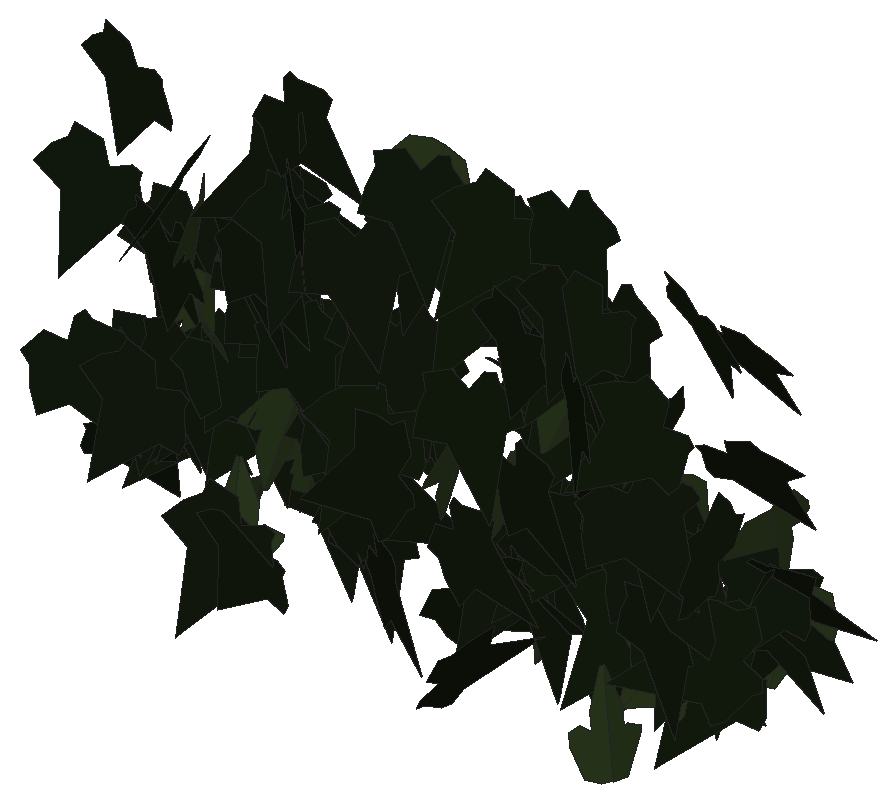
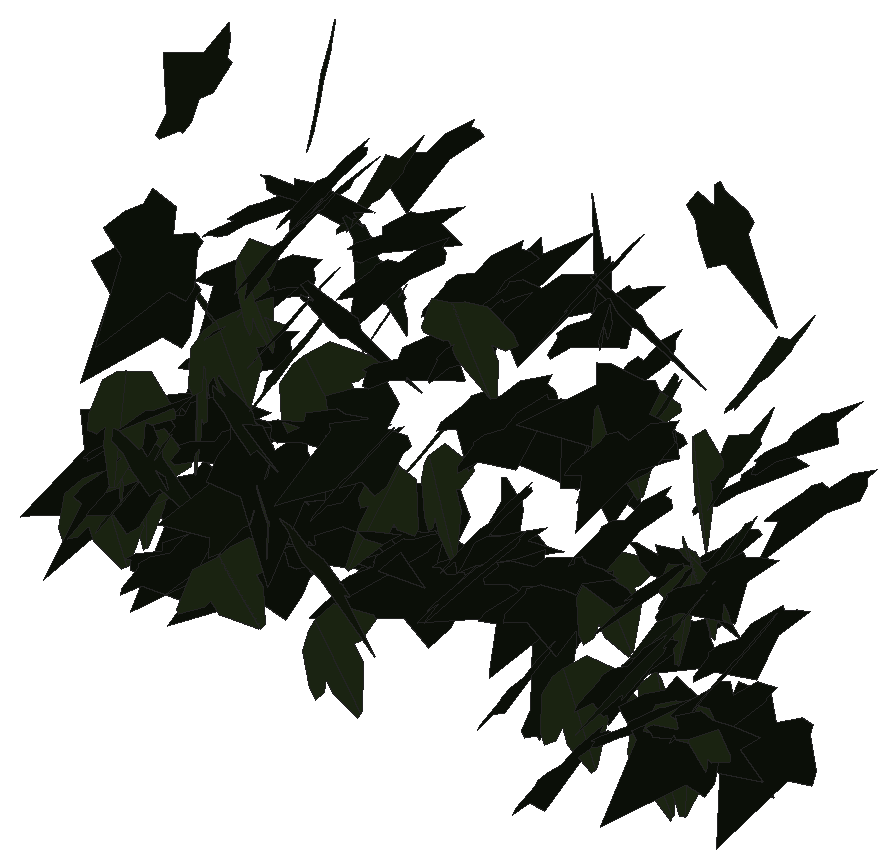
# SketchUp Ruby script. Lengths in inches.
U = 1.inch
M = Sketchup.active_model
def pt(a) = Geom::Point3d.new(a.map { |v| v * U })
def face(e, loops, mat)
  f = e.add_face(loops[0].map { |a| pt(a) })
  loops[1..].each { |l| e.add_face(l.map { |a| pt(a) }).erase! }
  f.material = f.back_material = mat if mat
  f
end
# faces: each face lists its corners as indices into pts; further lists are holes
def faces(e, pts, list, mat = nil) = list.each { |f| face(e, (f[0].is_a?(Array) ? f : [f]).map { |l| l.map { |i| pts[i] } }, mat) }
# xy, xz, yz: faces in a plane at the given z, y or x. An outline is a flat list of corners, or four numbers for a rectangle; further outlines are holes
def ring(l) = l.size == 4 ? [[l[0], l[1]], [l[2], l[1]], [l[2], l[3]], [l[0], l[3]]] : l.each_slice(2).to_a
def flat(e, list, mat, &to3) = list.each { |f| face(e, (f[0].is_a?(Array) ? f : [f]).map { |l| ring(l).map { |u, v| to3.(u, v) } }, mat) }
def xy(e, z, list, mat = nil) = flat(e, list, mat) { |x, y| [x, y, z] }
def xz(e, y, list, mat = nil) = flat(e, list, mat) { |x, z| [x, y, z] }
def yz(e, x, list, mat = nil) = flat(e, list, mat) { |y, z| [x, y, z] }
def lines(e, pts, list) = list.each { |a, b| e.add_line(pt(pts[a]), pt(pts[b])) }
# prism: a flat outline (further loops are holes) pulled along v
def prism(e, loops, v, mat = nil)
  f = face(e, loops, mat); d = Geom::Vector3d.new(v.map { |x| x * U })
  f.pushpull(f.normal.samedirection?(d) ? d.length : -d.length)
end
def box(e, o, s, mat = nil) = prism(e, [[o, [o[0] + s[0], o[1], o[2]], [o[0] + s[0], o[1] + s[1], o[2]], [o[0], o[1] + s[1], o[2]]]], [0, 0, s[2]], mat)
def at(x, y, z, deg = 0) = Geom::Transformation.translation(pt([x, y, z])) * Geom::Transformation.rotation(ORIGIN, Z_AXIS, deg.degrees)
def axes(o, x, y, z) = Geom::Transformation.new([*x, 0, *y, 0, *z, 0, *pt(o).to_a, 1])
def part(name) = M.definitions.add(name)
# library, detail: a bought-in or finely detailed component or shape, given as its bounding box
def library(name, o, s) = part(name).tap { |d| box(d.entities, o, s) }
def detail(e, o, s) = box(e.add_group.entities, o, s)
def put(e, d, t, mat = nil) = e.add_instance(d, t).tap { |i| i.material = mat if mat }
def group(e, t, mat = nil) = e.add_group.tap { |g| g.transformation = t; g.material = mat if mat }.entities
root = M.entities
M.materials.add("efeu1").color = [18, 25, 13]
M.materials.add("efeu2").color = [43, 57, 29]
c1 = part("ivyleaf_9")
p = [[1.54,2.16,1.25],[1.36,2.04,1.19],[-0.21,0.99,0.68],[-0.71,1.11,0.82],[-0.85,0.86,0.67],[-0.8,0.17,0.21],
  [-0.9,-0.01,0.1],[-0.67,-0.16,-0.02],[-0.08,-0.08,-0.05],[-0.03,-0.6,-0.4],[0.65,-0.88,-0.66],[0.83,-0.6,-0.49],
  [1.29,-0.42,-0.43],[1.8125,-0.07,-0.26],[1.21,0.44,0.15]]
faces(c1.entities,p,[[0,1,2,3,4,5,6,7,8,9,10,11,12,13,14]],"efeu1")
c2 = part("ivyleaf_10")
p = [[0,0.5,-0.03],[-0.0625,2.02,-0.43],[-0.19,2.01,-0.46],[-0.54,1.05,-0.29],[-0.52,0.625,-0.18],[-0.83,0.76,-0.28],
  [-1.16,0.64,-0.33],[-1.15,0.33,-0.24],[-0.77,-0.39,0.02],[-0.3,-0.51,0.16],[0.04,-0.48,0.23],[-0.02,2.01,-0.4375],
  [-0.06,2.01,-0.43],[0.04,-0.49,0.23],[0.67,-0.49,0.14],[1.38,0.36,-0.2],[1.375,0.51,-0.24],[0.81,0.65,-0.19],
  [0.62,0.59,-0.15],[0.6,1.09,-0.28],[0.5,1.23,-0.31]]
faces(c2.entities,p,[[0,1,2,3,4,5,6,7,8,9,10],[11,12,0,13,14,15,16,17,18,19,20]],"efeu2")
put(root,c1,axes([29.21,220.93,249.09],[0.38995,0.30515,-0.06943],[-0.05603,-0.04106,-0.49515],[-0.30789,0.39395,0.00217]))
put(root,c1,axes([29.23,220.59,252.55],[-0.16358,-0.44301,0.16426],[-0.00318,-0.17279,-0.46919],[0.47247,-0.15454,0.05372]))
put(root,c1,axes([29.22,221.13,253.58],[-0.03475,-0.39781,0.3009],[0.08116,-0.30212,-0.39005],[0.49214,0.02173,0.08557]))
put(root,c1,axes([29.36,221.97,251.31],[-0.15964,-0.47334,0.02147],[-0.00888,-0.01966,-0.49953],[0.47375,-0.15987,-0.00213]))
put(root,c1,axes([29.66,221.94,249.32],[-0.4551,-0.20171,0.04684],[-0.04917,-0.00462,-0.49756],[0.20116,-0.45748,-0.01563]))
put(root,c2,axes([29.69,221.88,249.35],[-0.49291,0.00458,0.08381],[-0.08393,-0.02123,-0.49245],[-0.00095,-0.49953,0.0217]))
put(root,c1,axes([29.5,221.12,250.18],[-0.07345,-0.49439,0.01348],[-0.0043,-0.01299,-0.49981],[0.49456,-0.07354,-0.00234]))
put(root,c1,axes([29.4,221.29,250.07],[0.20532,-0.45347,-0.04697],[-0.00661,0.04855,-0.49759],[0.45585,0.20495,0.01394]))
put(root,c1,axes([29.46,221.38,249.5625],[0.14125,-0.2738,-0.39381],[-0.04334,0.40156,-0.29473],[0.47767,0.1174,0.08971]))
put(root,c1,axes([29.46,221.49,251.3125],[0.2592,-0.42737,-0.01299],[-0.00599,0.01156,-0.49983],[0.42752,0.25927,0.00088]))
put(root,c1,axes([29.68,221.79,249.27],[0.47958,0.1413,0.00649],[-0.00505,0.04001,-0.49837],[-0.14136,0.47795,0.0398]))
put(root,c1,axes([29.8,219.25,251.125],[0.145,-0.39309,-0.27286],[0.02102,0.29007,-0.40671],[0.47805,0.10647,0.10064]))
put(root,c2,axes([29.99,221.26,250.9375],[0.42649,-0.23283,0.11788],[0.0984,-0.0657,-0.4858],[0.24171,0.43758,-0.01022]))
put(root,c2,axes([30.15,221.04,252.18],[0.19519,-0.44786,-0.10639],[-0.00593,0.11311,-0.487],[0.46029,0.19137,0.03884]))
put(root,c1,axes([30.15,222.27,249.375],[-0.2499,-0.39832,0.16998],[0.02614,-0.20977,-0.45312],[0.43228,-0.21758,0.12567]))
put(root,c1,axes([30,221.96,250.23],[0.35827,-0.2888,-0.19555],[-0.07662,0.20833,-0.44803],[0.34026,0.35099,0.10502]))
put(root,c2,axes([30.35,221.02,250.66],[-0.40851,0.26262,0.11896],[-0.11164,0.04613,-0.48519],[-0.26582,-0.42297,0.02095]))
put(root,c1,axes([30.03,220.67,251.87],[0.04267,-0.39306,0.30608],[0.10709,-0.29278,-0.39091],[0.48653,0.09892,0.0592]))
put(root,c1,axes([30.3,220.68,250.7],[0.0676,-0.49216,-0.05663],[-0.01008,0.05578,-0.49678],[0.49531,0.0683,-0.00238]))
put(root,c2,axes([30.63,221.4,248.61],[0.10762,-0.47372,0.11835],[0.02007,-0.11679,-0.48575],[0.48787,0.1093,-0.00613]))
put(root,c1,axes([30.49,221.88,249.82],[0.04318,-0.49066,-0.08596],[-0.0039,0.08595,-0.49254],[0.49812,0.04321,0.0036]))
put(root,c1,axes([30.84,220.83,250.6],[-0.48961,-0.07906,-0.0635],[0.06396,0.0022,-0.49589],[0.07869,-0.4937,0.00796]))
put(root,c1,axes([30.52,220.92,250.62],[0.25459,-0.35078,-0.24927],[0.02231,0.29999,-0.39938],[0.42975,0.19224,0.1684]))
put(root,c1,axes([30.75,221.57,252.41],[0.04534,-0.39982,-0.2968],[-0.01554,0.29674,-0.40212],[0.4977,0.04568,0.01448]))
put(root,c1,axes([30.91,219.31,250.92],[-0.21883,-0.38989,0.22382],[-0.02156,-0.23955,-0.43835],[0.44905,-0.2015,0.08803]))
put(root,c2,axes([30.96,220.68,248.33],[0.48743,-0.04738,0.10083],[-0.09416,0.06665,0.48651],[-0.05955,-0.49327,0.05605]))
put(root,c1,axes([30.95,221.37,251.27],[0.0906,-0.46973,-0.14542],[-0.01438,0.14528,-0.47821],[0.49151,0.09084,0.01282]))
put(root,c2,axes([31.21,221.98,249.32],[-0.11024,-0.4731,0.11843],[-0.00001,-0.12141,-0.48503],[0.4877,-0.10694,0.02676]))
put(root,c1,axes([31,221.19,251.98],[0.03372,-0.48274,-0.1258],[-0.02637,0.12418,-0.48361],[0.49816,0.03925,-0.01709]))
put(root,c2,axes([31.29,220.95,252.36],[-0.10922,-0.48607,0.04254],[-0.01699,-0.03977,-0.49813],[0.48763,-0.11025,-0.00783]))
put(root,c1,axes([31.04,222.36,248.59],[0.08334,-0.49281,-0.0139],[-0.00136,0.01387,-0.49981],[0.493,0.08334,0.00098]))
put(root,c1,axes([30.93,221.0625,252.5],[0.16379,0.04482,-0.47028],[0.24795,0.41552,0.12596],[0.40211,-0.27447,0.11388]))
put(root,c1,axes([31.09,220.76,252.15],[0.23479,-0.43206,0.09053],[0.03812,-0.08231,-0.4917],[0.4398,0.23779,-0.00571]))
put(root,c1,axes([31.56,218.98,253.93],[-0.31276,0.3652,-0.13716],[0.08032,-0.11175,-0.48069],[-0.38175,-0.32271,0.01124]))
put(root,c1,axes([31.42,220.17,248.97],[-0.20972,-0.42759,0.15228],[-0.05879,-0.14074,-0.47617],[0.45007,-0.21763,0.00875]))
put(root,c2,axes([31.45,221.09,250.16],[-0.07619,-0.45606,0.19027],[0.05657,-0.1993,-0.45506],[0.49091,-0.04781,0.08197]))
put(root,c1,axes([31.78,220.58,253.47],[-0.4591,0.16955,0.10239],[-0.09907,0.02725,-0.48933],[-0.17151,-0.46959,0.00858]))
put(root,c1,axes([31.52,220.36,252.62],[0.19122,-0.39391,-0.24139],[-0.08314,0.22765,-0.43734],[0.45445,0.2074,0.02156]))
put(root,c1,axes([31.66,222.02,250.72],[-0.284,-0.3953,-0.11438],[0.12868,0.0467,-0.4809],[0.39088,-0.30258,0.07521]))
put(root,c1,axes([31.5625,220.88,254.04],[0.29797,-0.32374,-0.23749],[-0.07733,0.24394,-0.42955],[0.394,0.29272,0.09531]))
put(root,c1,axes([31.69,221.53,250.18],[-0.17455,-0.43661,-0.17002],[0.04447,0.16518,-0.46983],[0.46643,-0.17913,-0.01884]))
put(root,c1,axes([31.66,220.19,248.74],[-0.14179,-0.3211,0.35607],[0.08349,-0.38218,-0.3114],[0.47215,-0.02885,0.162]))
put(root,c1,axes([31.93,221.54,250.04],[0.02012,-0.3952,-0.30563],[0.04905,0.30596,-0.3924],[0.49718,-0.0142,0.05108]))
put(root,c1,axes([31.84,221.55,248.78],[0.0941,-0.26061,0.41621],[0.15635,-0.38583,-0.27693],[0.46551,0.18227,0.00888]))
put(root,c1,axes([32.1,220.5,253.05],[-0.13153,-0.47649,0.07521],[-0.01856,-0.07289,-0.49431],[0.48203,-0.13282,0.00148]))
put(root,c1,axes([31.96,220.55,251.49],[-0.16432,-0.18296,-0.43534],[0.41457,0.16483,-0.22575],[0.22612,-0.43515,0.09753]))
put(root,c1,axes([32.19,220.2,252.9],[-0.03375,0.062,0.49499],[0.11023,-0.48293,0.06801],[0.48653,0.11371,0.01893]))
put(root,c1,axes([32.3,221.47,248.87],[0.1202,-0.48356,0.04149],[0.00684,-0.04105,-0.49826],[0.48529,0.12035,-0.00325]))
put(root,c1,axes([32.3,222.1875,250.59],[0.19231,-0.44588,-0.11919],[0.03219,0.14176,-0.4784],[0.46041,0.17633,0.08323]))
put(root,c1,axes([32.46,221.84,250.93],[0.14967,-0.47524,-0.0418],[0.0054,0.04549,-0.4979],[0.47704,0.14859,0.01875]))
put(root,c1,axes([32.92,221.61,250.28],[-0.33707,-0.30441,0.20909],[-0.06938,-0.22585,-0.44066],[0.36273,-0.32607,0.11002]))
put(root,c2,axes([32.87,221.82,253.35],[0.48617,0.01908,-0.11523],[-0.11589,0.01708,-0.48609],[-0.01461,0.49934,0.02103]))
put(root,c1,axes([32.79,221.16,251.7],[-0.05047,-0.49737,0.00893],[-0.00216,-0.00876,-0.49992],[0.49744,-0.0505,-0.00126]))
put(root,c1,axes([32.76,220.65,249.7],[0.07449,-0.02743,-0.49366],[0.15635,0.47492,-0.00279],[0.46905,-0.15395,0.07933]))
put(root,c1,axes([32.93,220.36,253.04],[-0.11873,-0.41975,-0.24435],[0.07975,0.23129,-0.43606],[0.47911,-0.14252,0.01203]))
put(root,c1,axes([33.05,221.5,252.92],[-0.04662,-0.48211,0.12409],[-0.02844,-0.12185,-0.48409],[0.49701,-0.05219,-0.01606]))
put(root,c1,axes([33.14,221.24,253.5625],[-0.0217,-0.49082,-0.09288],[-0.00599,0.09322,-0.4912],[0.49949,-0.0202,-0.00992]))
put(root,c1,axes([33.17,220.8,251.79],[-0.02376,-0.45354,-0.20914],[0.0415,0.20686,-0.45331],[0.49771,-0.0389,0.02781]))
put(root,c1,axes([33.43,220.25,251.04],[-0.37501,-0.33064,-0.00649],[0.00466,0.00454,-0.49996],[0.33068,-0.37504,-0.00032]))
put(root,c1,axes([33.87,221.63,252.42],[-0.26422,-0.41147,0.10432],[-0.01642,-0.11287,-0.48682],[0.42417,-0.26068,0.04613]))
put(root,c2,axes([33.93,220.94,250.59],[0.11476,-0.48662,0.00577],[0.00035,-0.00585,-0.49997],[0.48665,0.11475,-0.001]))
put(root,c1,axes([33.68,219.84,249.48],[-0.00478,0.01268,-0.49982],[0.49997,0.00282,-0.00471],[0.0027,-0.49983,-0.0127]))
put(root,c1,axes([34.23,221.26,253.31],[0.08681,-0.44766,-0.20509],[0.03196,0.21293,-0.45126],[0.49137,0.06524,0.06559]))
put(root,c1,axes([34.22,221.56,251.35],[0.49878,-0.00333,0.03481],[0.03468,0.11031,-0.48645],[-0.00444,0.48767,0.11027]))
put(root,c1,axes([34.51,221.11,253.53],[-0.2849,-0.3775,0.16226],[-0.0426,-0.16925,-0.46855],[0.40868,-0.2808,0.06428]))
put(root,c1,axes([34.34,221.86,250.95],[0.10015,-0.48708,0.05214],[0.00665,-0.05186,-0.49726],[0.48982,0.10029,-0.00391]))
put(root,c2,axes([34.56,220.95,250.24],[-0.03044,-0.34577,-0.35988],[0.11041,0.34695,-0.34269],[0.48671,-0.10033,0.05523]))
put(root,c1,axes([34.36,220.51,249.1],[0.02381,0.07549,-0.4937],[0.19024,0.45562,0.07884],[0.46178,-0.1916,-0.00702]))
put(root,c1,axes([34.64,221.11,249.3],[-0.22202,-0.41506,0.16861],[-0.04736,-0.16538,-0.46947],[0.44549,-0.22443,0.03413]))
put(root,c2,axes([34.72,221.9,248.68],[0.02273,-0.47514,0.15401],[-0.01257,-0.15467,-0.47531],[0.49932,0.01774,-0.01897]))
put(root,c1,axes([35.04,221.78,249.625],[-0.30409,0.35256,0.18229],[-0.13128,0.12738,-0.46534],[-0.37456,-0.33087,0.0151]))
put(root,c1,axes([34.85,218.64,251.52],[-0.15369,-0.16433,0.44652],[-0.21674,-0.39354,-0.21943],[0.42356,-0.261,0.04973]))
put(root,c1,axes([35.12,221.51,252.6],[-0.46747,0.12225,0.12855],[-0.124,0.03391,-0.48319],[-0.12685,-0.48364,-0.00138]))
put(root,c1,axes([35.02,221.64,249.66],[-0.3741,-0.31618,0.10039],[-0.03406,-0.1139,-0.48566],[0.32998,-0.37021,0.06368]))
put(root,c1,axes([35.35,221.23,249.87],[-0.00754,0.02933,-0.49908],[-0.33103,-0.37434,-0.017],[-0.37465,0.33017,0.02506]))
put(root,c1,axes([34.85,219.75,250.3],[0.33383,-0.27333,-0.25269],[-0.11519,0.24691,-0.41925],[0.35397,0.33812,0.10188]))
put(root,c1,axes([35.125,221.72,251.2],[-0.38802,-0.31476,0.0192],[0.0256,-0.06179,-0.49551],[0.3143,-0.38355,0.06407]))
put(root,c1,axes([34.88,221.26,249.01],[0.12226,-0.46589,0.13416],[0.03154,-0.13043,-0.48166],[0.48379,0.12624,-0.0025]))
put(root,c1,axes([35.01,219.31,248.6875],[0.21084,0.21838,0.39731],[0.20931,0.3418,-0.29894],[-0.40217,0.29238,0.05271]))
put(root,c2,axes([35.25,221.45,251.63],[-0.20316,-0.40663,0.20827],[-0.05677,-0.2037,-0.45308],[0.45332,-0.20775,0.0366]))
put(root,c1,axes([35.63,219.87,252.26],[-0.32184,0.21914,-0.31369],[-0.255,0.18278,0.38932],[0.2853,0.41057,-0.00589]))
put(root,c1,axes([35.64,221.68,250.59],[0.05845,0.49587,-0.02646],[-0.00218,-0.02639,-0.4993],[-0.49657,0.05849,-0.00092]))
put(root,c1,axes([35.375,221.08,253.92],[0.1548,-0.46571,-0.09567],[-0.0194,0.09434,-0.49064],[0.47504,0.15561,0.01114]))
put(root,c2,axes([35.52,221.99,249.96],[-0.16429,0.12612,-0.45508],[0.14907,-0.44335,-0.17669],[-0.44809,-0.19374,0.10808]))
put(root,c1,axes([35.63,221.41,252.1875],[0.07376,-0.47402,0.14096],[0.03381,-0.13735,-0.47958],[0.49337,0.08028,0.01179]))
put(root,c1,axes([35.6875,219.78,251.36],[0.30031,-0.34824,-0.19633],[-0.12618,0.15043,-0.45984],[0.37933,0.32573,0.00247]))
put(root,c1,axes([35.68,219.9,253.03],[-0.02077,-0.39149,0.31033],[0.0929,-0.30821,-0.38259],[0.49085,0.04177,0.08554]))
put(root,c1,axes([35.64,221.36,251.68],[0.16423,-0.46033,0.10549],[0.03888,-0.09812,-0.48873],[0.47066,0.16873,0.00357]))
put(root,c1,axes([36.19,221.77,251.11],[-0.43043,0.23391,-0.10008],[0.06885,-0.08224,-0.48836],[-0.24493,-0.43419,0.03858]))
put(root,c1,axes([35.88,220.63,253.16],[-0.08579,-0.43179,0.23706],[0.03439,-0.2453,-0.43434],[0.49138,-0.05822,0.07178]))
put(root,c1,axes([35.77,222.04,250.1875],[0.38677,-0.29136,0.12458],[0.1285,-0.03547,-0.4819],[0.28965,0.40479,0.04744]))
put(root,c1,axes([35.95,218.59,252.95],[0.02936,-0.48778,-0.10586],[0.00683,0.10643,-0.48849],[0.49909,0.02724,0.01291]))
put(root,c1,axes([35.97,221.12,252.9375],[0.17659,-0.46299,-0.06679],[-0.01976,0.06394,-0.4955],[0.46736,0.17764,0.00428]))
put(root,c1,axes([36.27,220.46,253.22],[-0.45164,-0.20362,-0.06754],[0.10092,-0.06276,-0.48567],[0.18931,-0.45233,0.09779]))
put(root,c2,axes([36.3,221.7,248.95],[0.23409,0.38896,-0.20955],[-0.1415,-0.15865,-0.45256],[-0.41854,0.27118,0.03581]))
put(root,c1,axes([36.49,221.01,249.41],[-0.43091,-0.25116,0.03518],[-0.03236,-0.01433,-0.49875],[0.25154,-0.4321,-0.0039]))
put(root,c1,axes([36.27,220.85,248.84],[0.03976,-0.02722,-0.49767],[0.00935,0.49921,-0.02655],[0.49833,-0.0072,0.04021]))
put(root,c2,axes([36.94,219.8,248.1875],[0.00255,0.4812,-0.1358],[-0.01797,0.1358,0.48087],[0.49967,0.00243,0.01799]))
put(root,c1,axes([36.87,221.13,250.1],[-0.27443,-0.41772,0.01417],[0.05633,-0.05377,-0.4939],[0.41415,-0.26948,0.07657]))
put(root,c2,axes([36.9,220.55,251.92],[0.17293,-0.45376,0.11913],[0.0434,-0.11095,-0.4856],[0.46713,0.17829,0.00101]))
put(root,c2,axes([37.11,220.64,249.17],[0.40393,-0.13997,-0.25933],[-0.25082,0.06768,-0.42721],[0.15469,0.47521,-0.01553]))
put(root,c1,axes([36.84,221.98,249.07],[-0.068,-0.49482,-0.02303],[0.00282,0.02286,-0.49947],[0.49535,-0.06806,-0.00032]))
put(root,c2,axes([37.08,220.77,251.13],[-0.1945,-0.42494,0.17775],[0.04898,-0.21093,-0.45068],[0.45801,-0.1579,0.12368]))
put(root,c1,axes([37.01,220.93,249.03],[0.48018,0.1387,0.01364],[0.01309,0.00383,-0.49981],[-0.13875,0.48036,0.00005]))
put(root,c1,axes([37.12,220.53,251.24],[-0.03009,-0.49606,0.05498],[-0.00233,-0.05494,-0.49697],[0.49909,-0.03016,0.00099]))
put(root,c1,axes([37.35,220.18,252.32],[-0.31378,-0.27681,0.27371],[-0.07941,-0.29864,-0.39307],[0.3811,-0.29015,0.14345]))
put(root,c1,axes([37.32,221.48,248.72],[-0.33277,-0.35586,0.11237],[-0.00829,-0.14348,-0.4789],[0.37309,-0.32059,0.08959]))
put(root,c2,axes([37.3,220.875,250.6],[0.28308,-0.37631,-0.16809],[0.01097,0.21072,-0.45329],[0.412,0.25295,0.12756]))
put(root,c1,axes([37.17,221.61,252.77],[0.48155,0.08524,-0.10414],[-0.10886,0.01929,-0.48762],[-0.07911,0.4923,0.03713]))
put(root,c1,axes([37.66,221.64,250.06],[-0.41606,0.24934,-0.12133],[0.05987,-0.13285,-0.4783],[-0.27075,-0.41253,0.0807]))
put(root,c1,axes([37.27,219.8,251.57],[0.0201,-0.36499,-0.34114],[0.10537,0.33683,-0.35418],[0.48836,-0.05766,0.09046]))
put(root,c1,axes([37.28,220.15,250.72],[0.07317,-0.38338,-0.31251],[0.05785,0.32038,-0.37949],[0.49122,0.01937,0.09124]))
put(root,c1,axes([37.31,218.73,253.43],[0.07498,-0.02511,-0.49371],[0.45347,-0.19534,0.0788],[-0.19684,-0.45958,-0.00652]))
put(root,c1,axes([37.67,220.67,249.92],[-0.31202,-0.39067,-0.0046],[0.00317,0.00335,-0.49998],[0.39068,-0.31204,0.00039]))
put(root,c2,axes([37.73,221.68,250.625],[-0.11494,-0.46478,-0.14413],[0.04224,0.138,-0.47872],[0.48477,-0.12222,0.00754]))
put(root,c2,axes([37.73,221.32,249.66],[-0.0067,-0.49678,-0.05621],[0.04629,0.05536,-0.49476],[0.49781,-0.01183,0.04526]))
put(root,c2,axes([37.81,221.99,249.48],[-0.34402,-0.33047,0.14979],[0.00679,-0.21225,-0.45266],[0.36277,-0.30942,0.15053]))
put(root,c1,axes([37.59,219.91,250.12],[0.1206,-0.46986,0.12121],[0.0305,-0.11731,-0.48509],[0.48428,0.1244,0.00036]))
put(root,c1,axes([37.58,221.65,249.61],[0.30076,-0.38428,-0.10896],[-0.02897,0.11505,-0.48572],[0.39838,0.29848,0.04694]))
put(root,c1,axes([37.74,221.67,249.57],[0.15868,-0.22398,-0.41792],[-0.1281,0.40406,-0.26519],[0.45652,0.19123,0.07085]))
put(root,c1,axes([37.86,221.62,250.01],[-0.19543,-0.41386,0.20132],[-0.04245,-0.20157,-0.45559],[0.45826,-0.19517,0.04366]))
put(root,c1,axes([37.58,221.65,249.79],[0.45712,0.05287,0.19556],[0.19309,0.03228,-0.46008],[-0.06127,0.49615,0.00909]))
put(root,c1,axes([37.74,220.99,251.75],[0.4775,0.14764,-0.01381],[-0.01315,-0.00424,-0.49981],[-0.14771,0.47769,-0.00017]))
put(root,c1,axes([38.29,220.38,249.625],[-0.39637,-0.03372,0.30291],[-0.28019,-0.15524,-0.38392],[0.11994,-0.47409,0.10417]))
put(root,c1,axes([38.4,219.86,251.14],[-0.31854,0.31968,0.21527],[-0.14831,0.1561,-0.45126],[-0.35572,-0.35134,-0.00462]))
put(root,c1,axes([37.78,220.36,253.8],[0.13059,-0.35876,0.32286],[0.18791,-0.27029,-0.37634],[0.44456,0.21963,0.06424]))
